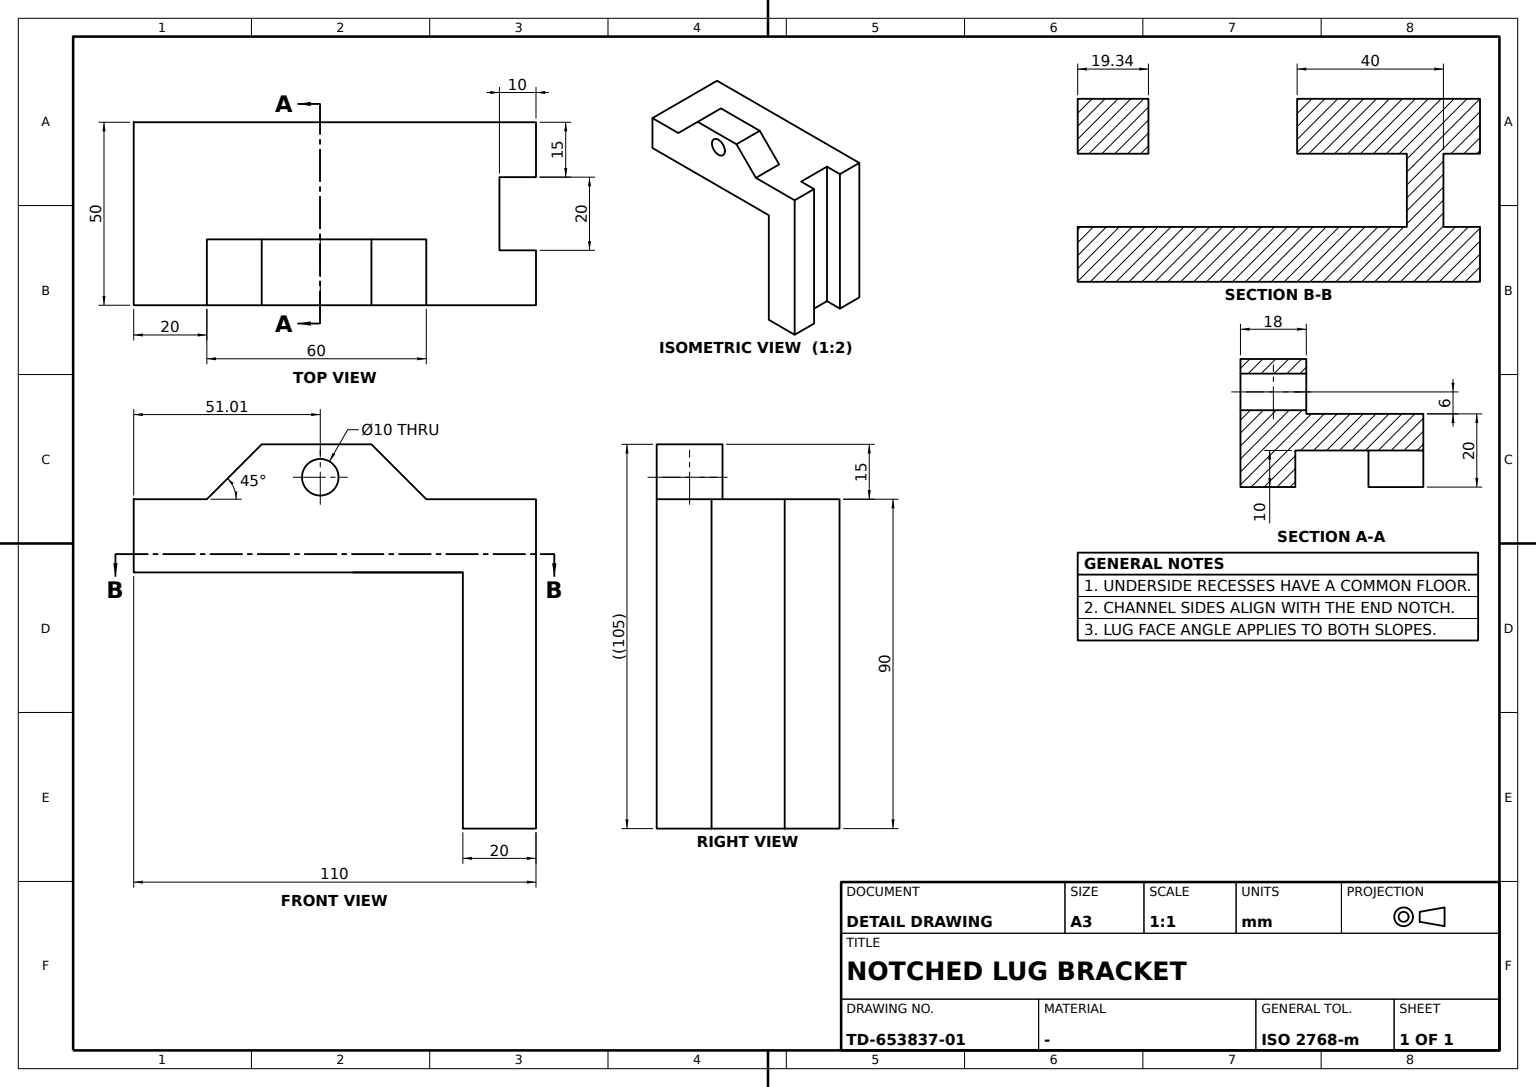
ISO-10303-21;
HEADER;
FILE_DESCRIPTION((''),'2;1');
FILE_NAME('','',(''),(''),'','','');
FILE_SCHEMA(('AUTOMOTIVE_DESIGN'));
ENDSEC;
DATA;
#1=APPLICATION_CONTEXT('');
#2=PRODUCT_CONTEXT('',#1,'mechanical');
#3=PRODUCT('','','',(#2));
#4=PRODUCT_DEFINITION_FORMATION('','',#3);
#5=PRODUCT_DEFINITION_CONTEXT('',#1,'design');
#6=PRODUCT_DEFINITION('','',#4,#5);
#7=PRODUCT_DEFINITION_SHAPE('','',#6);
#8=(LENGTH_UNIT()NAMED_UNIT(*)SI_UNIT(.MILLI.,.METRE.));
#9=(NAMED_UNIT(*)PLANE_ANGLE_UNIT()SI_UNIT($,.RADIAN.));
#10=(NAMED_UNIT(*)SI_UNIT($,.STERADIAN.)SOLID_ANGLE_UNIT());
#11=UNCERTAINTY_MEASURE_WITH_UNIT(LENGTH_MEASURE(1.E-05),#8,'distance_accuracy_value','');
#12=(GEOMETRIC_REPRESENTATION_CONTEXT(3)GLOBAL_UNCERTAINTY_ASSIGNED_CONTEXT((#11))GLOBAL_UNIT_ASSIGNED_CONTEXT((#8,#9,#10))REPRESENTATION_CONTEXT('',''));
#13=CARTESIAN_POINT('',(-33.986597,-12.,6.));
#14=VERTEX_POINT('',#13);
#15=CARTESIAN_POINT('',(-33.986597,-30.,6.));
#16=VERTEX_POINT('',#15);
#17=CARTESIAN_POINT('',(-33.986597,-21.66,6.));
#18=DIRECTION('',(0.,-1.,0.));
#19=VECTOR('',#18,1000.);
#20=LINE('',#17,#19);
#21=EDGE_CURVE('',#14,#16,#20,.T.);
#22=ORIENTED_EDGE('',*,*,#21,.T.);
#23=CARTESIAN_POINT('',(-43.986597,-30.,6.));
#24=VERTEX_POINT('',#23);
#25=CARTESIAN_POINT('',(-38.986597,-30.,6.));
#26=DIRECTION('',(0.,0.,1.));
#27=AXIS2_PLACEMENT_3D('',#25,#18,#26);
#28=CIRCLE('',#27,5.);
#29=EDGE_CURVE('',#16,#24,#28,.T.);
#30=ORIENTED_EDGE('',*,*,#29,.T.);
#31=CARTESIAN_POINT('',(-43.986597,-12.,6.));
#32=VERTEX_POINT('',#31);
#33=CARTESIAN_POINT('',(-43.986597,-21.66,6.));
#34=LINE('',#33,#19);
#35=EDGE_CURVE('',#32,#24,#34,.T.);
#36=ORIENTED_EDGE('',*,*,#35,.F.);
#37=CARTESIAN_POINT('',(-38.986597,-12.,6.));
#38=DIRECTION('',(0.,1.,0.));
#39=DIRECTION('',(-1.,0.,0.));
#40=AXIS2_PLACEMENT_3D('',#37,#38,#39);
#41=CIRCLE('',#40,5.);
#42=EDGE_CURVE('',#32,#14,#41,.T.);
#43=ORIENTED_EDGE('',*,*,#42,.T.);
#44=EDGE_LOOP('',(#22,#30,#36,#43));
#45=FACE_OUTER_BOUND('',#44,.T.);
#46=CARTESIAN_POINT('',(-38.986597,-21.66,6.));
#47=AXIS2_PLACEMENT_3D('',#46,#18,#39);
#48=CYLINDRICAL_SURFACE('',#47,5.);
#49=ADVANCED_FACE('',(#45),#48,.F.);
#50=CARTESIAN_POINT('',(-70.664001,5.,-20.));
#51=VERTEX_POINT('',#50);
#52=CARTESIAN_POINT('',(-90.,5.,-20.));
#53=VERTEX_POINT('',#52);
#54=CARTESIAN_POINT('',(-80.332001,5.,-20.));
#55=VECTOR('',#39,1000.);
#56=LINE('',#54,#55);
#57=EDGE_CURVE('',#51,#53,#56,.T.);
#58=ORIENTED_EDGE('',*,*,#57,.T.);
#59=CARTESIAN_POINT('',(-90.,20.,-20.));
#60=VERTEX_POINT('',#59);
#61=CARTESIAN_POINT('',(-90.,12.5,-20.));
#62=VECTOR('',#38,1000.);
#63=LINE('',#61,#62);
#64=EDGE_CURVE('',#53,#60,#63,.T.);
#65=ORIENTED_EDGE('',*,*,#64,.T.);
#66=CARTESIAN_POINT('',(-70.664001,20.,-20.));
#67=VERTEX_POINT('',#66);
#68=CARTESIAN_POINT('',(-80.332001,20.,-20.));
#69=LINE('',#68,#55);
#70=EDGE_CURVE('',#67,#60,#69,.T.);
#71=ORIENTED_EDGE('',*,*,#70,.F.);
#72=CARTESIAN_POINT('',(-70.664001,12.5,-20.));
#73=LINE('',#72,#19);
#74=EDGE_CURVE('',#67,#51,#73,.T.);
#75=ORIENTED_EDGE('',*,*,#74,.T.);
#76=EDGE_LOOP('',(#58,#65,#71,#75));
#77=FACE_OUTER_BOUND('',#76,.T.);
#78=CARTESIAN_POINT('',(0.,-15.,-20.));
#79=DIRECTION('',(0.,0.,-1.));
#80=AXIS2_PLACEMENT_3D('',#78,#79,#18);
#81=PLANE('',#80);
#82=ADVANCED_FACE('',(#77),#81,.T.);
#83=CARTESIAN_POINT('',(0.,-30.,-20.));
#84=VERTEX_POINT('',#83);
#85=VERTEX_POINT('',#78);
#86=CARTESIAN_POINT('',(0.,-22.5,-20.));
#87=LINE('',#86,#62);
#88=EDGE_CURVE('',#84,#85,#87,.T.);
#89=ORIENTED_EDGE('',*,*,#88,.T.);
#90=CARTESIAN_POINT('',(0.,-15.,-10.));
#91=VERTEX_POINT('',#90);
#92=CARTESIAN_POINT('',(0.,-15.,-15.));
#93=VECTOR('',#26,1000.);
#94=LINE('',#92,#93);
#95=EDGE_CURVE('',#85,#91,#94,.T.);
#96=ORIENTED_EDGE('',*,*,#95,.T.);
#97=CARTESIAN_POINT('',(0.,5.,-10.));
#98=VERTEX_POINT('',#97);
#99=CARTESIAN_POINT('',(0.,-5.,-10.));
#100=LINE('',#99,#62);
#101=EDGE_CURVE('',#91,#98,#100,.T.);
#102=ORIENTED_EDGE('',*,*,#101,.T.);
#103=CARTESIAN_POINT('',(0.,5.,-20.));
#104=VERTEX_POINT('',#103);
#105=CARTESIAN_POINT('',(0.,5.,-15.));
#106=VECTOR('',#79,1000.);
#107=LINE('',#105,#106);
#108=EDGE_CURVE('',#98,#104,#107,.T.);
#109=ORIENTED_EDGE('',*,*,#108,.T.);
#110=CARTESIAN_POINT('',(0.,20.,-20.));
#111=VERTEX_POINT('',#110);
#112=CARTESIAN_POINT('',(0.,12.5,-20.));
#113=LINE('',#112,#62);
#114=EDGE_CURVE('',#104,#111,#113,.T.);
#115=ORIENTED_EDGE('',*,*,#114,.T.);
#116=CARTESIAN_POINT('',(0.,20.,-90.));
#117=VERTEX_POINT('',#116);
#118=CARTESIAN_POINT('',(0.,20.,-55.));
#119=LINE('',#118,#106);
#120=EDGE_CURVE('',#111,#117,#119,.T.);
#121=ORIENTED_EDGE('',*,*,#120,.T.);
#122=CARTESIAN_POINT('',(0.,-30.,-90.));
#123=VERTEX_POINT('',#122);
#124=CARTESIAN_POINT('',(0.,-5.,-90.));
#125=LINE('',#124,#19);
#126=EDGE_CURVE('',#117,#123,#125,.T.);
#127=ORIENTED_EDGE('',*,*,#126,.T.);
#128=CARTESIAN_POINT('',(0.,-30.,-55.));
#129=LINE('',#128,#106);
#130=EDGE_CURVE('',#84,#123,#129,.T.);
#131=ORIENTED_EDGE('',*,*,#130,.F.);
#132=EDGE_LOOP('',(#89,#96,#102,#109,#115,#121,#127,#131));
#133=FACE_OUTER_BOUND('',#132,.T.);
#134=CARTESIAN_POINT('',(0.,0.,0.));
#135=DIRECTION('',(1.,0.,0.));
#136=AXIS2_PLACEMENT_3D('',#134,#135,#38);
#137=PLANE('',#136);
#138=ADVANCED_FACE('',(#133),#137,.F.);
#139=CARTESIAN_POINT('',(10.,5.,0.));
#140=VERTEX_POINT('',#139);
#141=CARTESIAN_POINT('',(10.,5.,-90.));
#142=VERTEX_POINT('',#141);
#143=CARTESIAN_POINT('',(10.,5.,-45.));
#144=LINE('',#143,#106);
#145=EDGE_CURVE('',#140,#142,#144,.T.);
#146=ORIENTED_EDGE('',*,*,#145,.F.);
#147=CARTESIAN_POINT('',(10.,-15.,0.));
#148=VERTEX_POINT('',#147);
#149=CARTESIAN_POINT('',(10.,-5.,0.));
#150=LINE('',#149,#62);
#151=EDGE_CURVE('',#148,#140,#150,.T.);
#152=ORIENTED_EDGE('',*,*,#151,.F.);
#153=CARTESIAN_POINT('',(10.,-15.,-90.));
#154=VERTEX_POINT('',#153);
#155=CARTESIAN_POINT('',(10.,-15.,-45.));
#156=LINE('',#155,#106);
#157=EDGE_CURVE('',#148,#154,#156,.T.);
#158=ORIENTED_EDGE('',*,*,#157,.T.);
#159=CARTESIAN_POINT('',(10.,-5.,-90.));
#160=LINE('',#159,#62);
#161=EDGE_CURVE('',#154,#142,#160,.T.);
#162=ORIENTED_EDGE('',*,*,#161,.T.);
#163=EDGE_LOOP('',(#146,#152,#158,#162));
#164=FACE_OUTER_BOUND('',#163,.T.);
#165=AXIS2_PLACEMENT_3D('',#139,#135,#18);
#166=PLANE('',#165);
#167=ADVANCED_FACE('',(#164),#166,.T.);
#168=CARTESIAN_POINT('',(-30.,20.,-20.));
#169=VERTEX_POINT('',#168);
#170=CARTESIAN_POINT('',(-30.,5.,-20.));
#171=VERTEX_POINT('',#170);
#172=CARTESIAN_POINT('',(-30.,12.5,-20.));
#173=LINE('',#172,#19);
#174=EDGE_CURVE('',#169,#171,#173,.T.);
#175=ORIENTED_EDGE('',*,*,#174,.T.);
#176=CARTESIAN_POINT('',(-30.,5.,-10.));
#177=VERTEX_POINT('',#176);
#178=CARTESIAN_POINT('',(-30.,5.,-15.));
#179=LINE('',#178,#93);
#180=EDGE_CURVE('',#171,#177,#179,.T.);
#181=ORIENTED_EDGE('',*,*,#180,.T.);
#182=CARTESIAN_POINT('',(-30.,20.,-10.));
#183=VERTEX_POINT('',#182);
#184=CARTESIAN_POINT('',(-30.,12.5,-10.));
#185=LINE('',#184,#19);
#186=EDGE_CURVE('',#183,#177,#185,.T.);
#187=ORIENTED_EDGE('',*,*,#186,.F.);
#188=CARTESIAN_POINT('',(-30.,20.,-15.));
#189=LINE('',#188,#106);
#190=EDGE_CURVE('',#183,#169,#189,.T.);
#191=ORIENTED_EDGE('',*,*,#190,.T.);
#192=EDGE_LOOP('',(#175,#181,#187,#191));
#193=FACE_OUTER_BOUND('',#192,.T.);
#194=AXIS2_PLACEMENT_3D('',#168,#135,#26);
#195=PLANE('',#194);
#196=ADVANCED_FACE('',(#193),#195,.F.);
#197=CARTESIAN_POINT('',(-70.,-30.,0.));
#198=VERTEX_POINT('',#197);
#199=CARTESIAN_POINT('',(-55.,-30.,15.));
#200=VERTEX_POINT('',#199);
#201=CARTESIAN_POINT('',(-62.5,-30.,7.5));
#202=DIRECTION('',(0.707106781,0.,0.707106781));
#203=VECTOR('',#202,1000.);
#204=LINE('',#201,#203);
#205=EDGE_CURVE('',#198,#200,#204,.T.);
#206=ORIENTED_EDGE('',*,*,#205,.T.);
#207=CARTESIAN_POINT('',(-55.,-12.,15.));
#208=VERTEX_POINT('',#207);
#209=CARTESIAN_POINT('',(-55.,-21.,15.));
#210=LINE('',#209,#19);
#211=EDGE_CURVE('',#208,#200,#210,.T.);
#212=ORIENTED_EDGE('',*,*,#211,.F.);
#213=CARTESIAN_POINT('',(-70.,-12.,0.));
#214=VERTEX_POINT('',#213);
#215=CARTESIAN_POINT('',(-62.5,-12.,7.5));
#216=DIRECTION('',(-0.707106781,0.,-0.707106781));
#217=VECTOR('',#216,1000.);
#218=LINE('',#215,#217);
#219=EDGE_CURVE('',#208,#214,#218,.T.);
#220=ORIENTED_EDGE('',*,*,#219,.T.);
#221=CARTESIAN_POINT('',(-70.,-21.,0.));
#222=LINE('',#221,#19);
#223=EDGE_CURVE('',#214,#198,#222,.T.);
#224=ORIENTED_EDGE('',*,*,#223,.T.);
#225=EDGE_LOOP('',(#206,#212,#220,#224));
#226=FACE_OUTER_BOUND('',#225,.T.);
#227=CARTESIAN_POINT('',(-70.,-33.6,0.));
#228=DIRECTION('',(0.707106781,0.,-0.707106781));
#229=AXIS2_PLACEMENT_3D('',#227,#228,#38);
#230=PLANE('',#229);
#231=ADVANCED_FACE('',(#226),#230,.F.);
#232=CARTESIAN_POINT('',(-90.,-30.,-20.));
#233=VERTEX_POINT('',#232);
#234=CARTESIAN_POINT('',(-90.,-15.,-20.));
#235=VERTEX_POINT('',#234);
#236=CARTESIAN_POINT('',(-90.,-22.5,-20.));
#237=LINE('',#236,#62);
#238=EDGE_CURVE('',#233,#235,#237,.T.);
#239=ORIENTED_EDGE('',*,*,#238,.F.);
#240=CARTESIAN_POINT('',(-90.,-30.,0.));
#241=VERTEX_POINT('',#240);
#242=CARTESIAN_POINT('',(-90.,-30.,-10.));
#243=LINE('',#242,#106);
#244=EDGE_CURVE('',#241,#233,#243,.T.);
#245=ORIENTED_EDGE('',*,*,#244,.F.);
#246=CARTESIAN_POINT('',(-90.,20.,0.));
#247=VERTEX_POINT('',#246);
#248=CARTESIAN_POINT('',(-90.,-5.,0.));
#249=LINE('',#248,#19);
#250=EDGE_CURVE('',#247,#241,#249,.T.);
#251=ORIENTED_EDGE('',*,*,#250,.F.);
#252=CARTESIAN_POINT('',(-90.,20.,-10.));
#253=LINE('',#252,#93);
#254=EDGE_CURVE('',#60,#247,#253,.T.);
#255=ORIENTED_EDGE('',*,*,#254,.F.);
#256=ORIENTED_EDGE('',*,*,#64,.F.);
#257=CARTESIAN_POINT('',(-90.,5.,-10.));
#258=VERTEX_POINT('',#257);
#259=CARTESIAN_POINT('',(-90.,5.,-15.));
#260=LINE('',#259,#106);
#261=EDGE_CURVE('',#258,#53,#260,.T.);
#262=ORIENTED_EDGE('',*,*,#261,.F.);
#263=CARTESIAN_POINT('',(-90.,-15.,-10.));
#264=VERTEX_POINT('',#263);
#265=CARTESIAN_POINT('',(-90.,-5.,-10.));
#266=LINE('',#265,#62);
#267=EDGE_CURVE('',#264,#258,#266,.T.);
#268=ORIENTED_EDGE('',*,*,#267,.F.);
#269=CARTESIAN_POINT('',(-90.,-15.,-15.));
#270=LINE('',#269,#93);
#271=EDGE_CURVE('',#235,#264,#270,.T.);
#272=ORIENTED_EDGE('',*,*,#271,.F.);
#273=EDGE_LOOP('',(#239,#245,#251,#255,#256,#262,#268,#272));
#274=FACE_OUTER_BOUND('',#273,.T.);
#275=CARTESIAN_POINT('',(-90.,0.,0.));
#276=AXIS2_PLACEMENT_3D('',#275,#135,#38);
#277=PLANE('',#276);
#278=ADVANCED_FACE('',(#274),#277,.F.);
#279=CARTESIAN_POINT('',(20.,-30.,0.));
#280=VERTEX_POINT('',#279);
#281=CARTESIAN_POINT('',(20.,-15.,0.));
#282=VERTEX_POINT('',#281);
#283=CARTESIAN_POINT('',(20.,-22.5,0.));
#284=LINE('',#283,#62);
#285=EDGE_CURVE('',#280,#282,#284,.T.);
#286=ORIENTED_EDGE('',*,*,#285,.F.);
#287=CARTESIAN_POINT('',(20.,-30.,-90.));
#288=VERTEX_POINT('',#287);
#289=CARTESIAN_POINT('',(20.,-30.,-45.));
#290=LINE('',#289,#106);
#291=EDGE_CURVE('',#280,#288,#290,.T.);
#292=ORIENTED_EDGE('',*,*,#291,.T.);
#293=CARTESIAN_POINT('',(20.,-15.,-90.));
#294=VERTEX_POINT('',#293);
#295=CARTESIAN_POINT('',(20.,-22.5,-90.));
#296=LINE('',#295,#62);
#297=EDGE_CURVE('',#288,#294,#296,.T.);
#298=ORIENTED_EDGE('',*,*,#297,.T.);
#299=CARTESIAN_POINT('',(20.,-15.,-45.));
#300=LINE('',#299,#106);
#301=EDGE_CURVE('',#282,#294,#300,.T.);
#302=ORIENTED_EDGE('',*,*,#301,.F.);
#303=EDGE_LOOP('',(#286,#292,#298,#302));
#304=FACE_OUTER_BOUND('',#303,.T.);
#305=AXIS2_PLACEMENT_3D('',#281,#135,#18);
#306=PLANE('',#305);
#307=ADVANCED_FACE('',(#304),#306,.T.);
#308=CARTESIAN_POINT('',(-45.,-15.,-20.));
#309=LINE('',#308,#55);
#310=EDGE_CURVE('',#85,#235,#309,.T.);
#311=ORIENTED_EDGE('',*,*,#310,.F.);
#312=ORIENTED_EDGE('',*,*,#88,.F.);
#313=CARTESIAN_POINT('',(-45.,-30.,-20.));
#314=LINE('',#313,#55);
#315=EDGE_CURVE('',#84,#233,#314,.T.);
#316=ORIENTED_EDGE('',*,*,#315,.T.);
#317=ORIENTED_EDGE('',*,*,#238,.T.);
#318=EDGE_LOOP('',(#311,#312,#316,#317));
#319=FACE_OUTER_BOUND('',#318,.T.);
#320=ADVANCED_FACE('',(#319),#81,.T.);
#321=CARTESIAN_POINT('',(20.,5.,0.));
#322=VERTEX_POINT('',#321);
#323=CARTESIAN_POINT('',(20.,5.,-90.));
#324=VERTEX_POINT('',#323);
#325=CARTESIAN_POINT('',(20.,5.,-45.));
#326=LINE('',#325,#106);
#327=EDGE_CURVE('',#322,#324,#326,.T.);
#328=ORIENTED_EDGE('',*,*,#327,.F.);
#329=CARTESIAN_POINT('',(15.,5.,0.));
#330=VECTOR('',#135,1000.);
#331=LINE('',#329,#330);
#332=EDGE_CURVE('',#140,#322,#331,.T.);
#333=ORIENTED_EDGE('',*,*,#332,.F.);
#334=ORIENTED_EDGE('',*,*,#145,.T.);
#335=CARTESIAN_POINT('',(15.,5.,-90.));
#336=LINE('',#335,#330);
#337=EDGE_CURVE('',#142,#324,#336,.T.);
#338=ORIENTED_EDGE('',*,*,#337,.T.);
#339=EDGE_LOOP('',(#328,#333,#334,#338));
#340=FACE_OUTER_BOUND('',#339,.T.);
#341=AXIS2_PLACEMENT_3D('',#103,#18,#26);
#342=PLANE('',#341);
#343=ADVANCED_FACE('',(#340),#342,.T.);
#344=CARTESIAN_POINT('',(-25.,-30.,15.));
#345=VERTEX_POINT('',#344);
#346=CARTESIAN_POINT('',(-25.,-12.,15.));
#347=VERTEX_POINT('',#346);
#348=CARTESIAN_POINT('',(-25.,-21.,15.));
#349=LINE('',#348,#62);
#350=EDGE_CURVE('',#345,#347,#349,.T.);
#351=ORIENTED_EDGE('',*,*,#350,.T.);
#352=CARTESIAN_POINT('',(-40.,-12.,15.));
#353=LINE('',#352,#55);
#354=EDGE_CURVE('',#347,#208,#353,.T.);
#355=ORIENTED_EDGE('',*,*,#354,.T.);
#356=ORIENTED_EDGE('',*,*,#211,.T.);
#357=CARTESIAN_POINT('',(-40.,-30.,15.));
#358=LINE('',#357,#330);
#359=EDGE_CURVE('',#200,#345,#358,.T.);
#360=ORIENTED_EDGE('',*,*,#359,.T.);
#361=EDGE_LOOP('',(#351,#355,#356,#360));
#362=FACE_OUTER_BOUND('',#361,.T.);
#363=CARTESIAN_POINT('',(0.,0.,15.));
#364=AXIS2_PLACEMENT_3D('',#363,#26,#135);
#365=PLANE('',#364);
#366=ADVANCED_FACE('',(#362),#365,.T.);
#367=ORIENTED_EDGE('',*,*,#180,.F.);
#368=CARTESIAN_POINT('',(-15.,5.,-20.));
#369=LINE('',#368,#55);
#370=EDGE_CURVE('',#104,#171,#369,.T.);
#371=ORIENTED_EDGE('',*,*,#370,.F.);
#372=ORIENTED_EDGE('',*,*,#108,.F.);
#373=CARTESIAN_POINT('',(-15.,5.,-10.));
#374=LINE('',#373,#55);
#375=EDGE_CURVE('',#98,#177,#374,.T.);
#376=ORIENTED_EDGE('',*,*,#375,.T.);
#377=EDGE_LOOP('',(#367,#371,#372,#376));
#378=FACE_OUTER_BOUND('',#377,.T.);
#379=ADVANCED_FACE('',(#378),#342,.T.);
#380=CARTESIAN_POINT('',(20.,20.,-90.));
#381=VERTEX_POINT('',#380);
#382=CARTESIAN_POINT('',(10.,20.,-90.));
#383=LINE('',#382,#55);
#384=EDGE_CURVE('',#381,#117,#383,.T.);
#385=ORIENTED_EDGE('',*,*,#384,.F.);
#386=CARTESIAN_POINT('',(20.,12.5,-90.));
#387=LINE('',#386,#62);
#388=EDGE_CURVE('',#324,#381,#387,.T.);
#389=ORIENTED_EDGE('',*,*,#388,.F.);
#390=ORIENTED_EDGE('',*,*,#337,.F.);
#391=ORIENTED_EDGE('',*,*,#161,.F.);
#392=CARTESIAN_POINT('',(15.,-15.,-90.));
#393=LINE('',#392,#55);
#394=EDGE_CURVE('',#294,#154,#393,.T.);
#395=ORIENTED_EDGE('',*,*,#394,.F.);
#396=ORIENTED_EDGE('',*,*,#297,.F.);
#397=CARTESIAN_POINT('',(10.,-30.,-90.));
#398=LINE('',#397,#330);
#399=EDGE_CURVE('',#123,#288,#398,.T.);
#400=ORIENTED_EDGE('',*,*,#399,.F.);
#401=ORIENTED_EDGE('',*,*,#126,.F.);
#402=EDGE_LOOP('',(#385,#389,#390,#391,#395,#396,#400,#401));
#403=FACE_OUTER_BOUND('',#402,.T.);
#404=CARTESIAN_POINT('',(0.,0.,-90.));
#405=AXIS2_PLACEMENT_3D('',#404,#26,#38);
#406=PLANE('',#405);
#407=ADVANCED_FACE('',(#403),#406,.F.);
#408=CARTESIAN_POINT('',(-10.,-12.,0.));
#409=VERTEX_POINT('',#408);
#410=CARTESIAN_POINT('',(-17.5,-12.,7.5));
#411=DIRECTION('',(-0.707106781,0.,0.707106781));
#412=VECTOR('',#411,1000.);
#413=LINE('',#410,#412);
#414=EDGE_CURVE('',#409,#347,#413,.T.);
#415=ORIENTED_EDGE('',*,*,#414,.T.);
#416=ORIENTED_EDGE('',*,*,#350,.F.);
#417=CARTESIAN_POINT('',(-10.,-30.,0.));
#418=VERTEX_POINT('',#417);
#419=CARTESIAN_POINT('',(-17.5,-30.,7.5));
#420=VECTOR('',#228,1000.);
#421=LINE('',#419,#420);
#422=EDGE_CURVE('',#345,#418,#421,.T.);
#423=ORIENTED_EDGE('',*,*,#422,.T.);
#424=CARTESIAN_POINT('',(-10.,-21.,0.));
#425=LINE('',#424,#62);
#426=EDGE_CURVE('',#418,#409,#425,.T.);
#427=ORIENTED_EDGE('',*,*,#426,.T.);
#428=EDGE_LOOP('',(#415,#416,#423,#427));
#429=FACE_OUTER_BOUND('',#428,.T.);
#430=CARTESIAN_POINT('',(-10.,-8.4,0.));
#431=AXIS2_PLACEMENT_3D('',#430,#216,#18);
#432=PLANE('',#431);
#433=ADVANCED_FACE('',(#429),#432,.F.);
#434=EDGE_CURVE('',#24,#16,#28,.T.);
#435=ORIENTED_EDGE('',*,*,#434,.T.);
#436=ORIENTED_EDGE('',*,*,#21,.F.);
#437=EDGE_CURVE('',#14,#32,#41,.T.);
#438=ORIENTED_EDGE('',*,*,#437,.T.);
#439=ORIENTED_EDGE('',*,*,#35,.T.);
#440=EDGE_LOOP('',(#435,#436,#438,#439));
#441=FACE_OUTER_BOUND('',#440,.T.);
#442=ADVANCED_FACE('',(#441),#48,.F.);
#443=CARTESIAN_POINT('',(-70.664001,20.,-10.));
#444=VERTEX_POINT('',#443);
#445=CARTESIAN_POINT('',(-50.332001,20.,-10.));
#446=LINE('',#445,#330);
#447=EDGE_CURVE('',#444,#183,#446,.T.);
#448=ORIENTED_EDGE('',*,*,#447,.T.);
#449=ORIENTED_EDGE('',*,*,#186,.T.);
#450=ORIENTED_EDGE('',*,*,#375,.F.);
#451=ORIENTED_EDGE('',*,*,#101,.F.);
#452=CARTESIAN_POINT('',(-45.,-15.,-10.));
#453=LINE('',#452,#55);
#454=EDGE_CURVE('',#91,#264,#453,.T.);
#455=ORIENTED_EDGE('',*,*,#454,.T.);
#456=ORIENTED_EDGE('',*,*,#267,.T.);
#457=CARTESIAN_POINT('',(-70.664001,5.,-10.));
#458=VERTEX_POINT('',#457);
#459=CARTESIAN_POINT('',(-80.332001,5.,-10.));
#460=LINE('',#459,#55);
#461=EDGE_CURVE('',#458,#258,#460,.T.);
#462=ORIENTED_EDGE('',*,*,#461,.F.);
#463=CARTESIAN_POINT('',(-70.664001,12.5,-10.));
#464=LINE('',#463,#19);
#465=EDGE_CURVE('',#444,#458,#464,.T.);
#466=ORIENTED_EDGE('',*,*,#465,.F.);
#467=EDGE_LOOP('',(#448,#449,#450,#451,#455,#456,#462,#466));
#468=FACE_OUTER_BOUND('',#467,.T.);
#469=AXIS2_PLACEMENT_3D('',#97,#79,#18);
#470=PLANE('',#469);
#471=ADVANCED_FACE('',(#468),#470,.T.);
#472=ORIENTED_EDGE('',*,*,#261,.T.);
#473=ORIENTED_EDGE('',*,*,#57,.F.);
#474=CARTESIAN_POINT('',(-70.664001,5.,-15.));
#475=LINE('',#474,#93);
#476=EDGE_CURVE('',#51,#458,#475,.T.);
#477=ORIENTED_EDGE('',*,*,#476,.T.);
#478=ORIENTED_EDGE('',*,*,#461,.T.);
#479=EDGE_LOOP('',(#472,#473,#477,#478));
#480=FACE_OUTER_BOUND('',#479,.T.);
#481=ADVANCED_FACE('',(#480),#342,.T.);
#482=ORIENTED_EDGE('',*,*,#254,.T.);
#483=CARTESIAN_POINT('',(20.,20.,0.));
#484=VERTEX_POINT('',#483);
#485=CARTESIAN_POINT('',(-35.,20.,0.));
#486=LINE('',#485,#55);
#487=EDGE_CURVE('',#484,#247,#486,.T.);
#488=ORIENTED_EDGE('',*,*,#487,.F.);
#489=CARTESIAN_POINT('',(20.,20.,-45.));
#490=LINE('',#489,#106);
#491=EDGE_CURVE('',#484,#381,#490,.T.);
#492=ORIENTED_EDGE('',*,*,#491,.T.);
#493=ORIENTED_EDGE('',*,*,#384,.T.);
#494=ORIENTED_EDGE('',*,*,#120,.F.);
#495=CARTESIAN_POINT('',(-15.,20.,-20.));
#496=LINE('',#495,#55);
#497=EDGE_CURVE('',#111,#169,#496,.T.);
#498=ORIENTED_EDGE('',*,*,#497,.T.);
#499=ORIENTED_EDGE('',*,*,#190,.F.);
#500=ORIENTED_EDGE('',*,*,#447,.F.);
#501=CARTESIAN_POINT('',(-70.664001,20.,-15.));
#502=LINE('',#501,#93);
#503=EDGE_CURVE('',#67,#444,#502,.T.);
#504=ORIENTED_EDGE('',*,*,#503,.F.);
#505=ORIENTED_EDGE('',*,*,#70,.T.);
#506=EDGE_LOOP('',(#482,#488,#492,#493,#494,#498,#499,#500,#504,#505));
#507=FACE_OUTER_BOUND('',#506,.T.);
#508=CARTESIAN_POINT('',(0.,20.,0.));
#509=AXIS2_PLACEMENT_3D('',#508,#38,#79);
#510=PLANE('',#509);
#511=ADVANCED_FACE('',(#507),#510,.T.);
#512=ORIENTED_EDGE('',*,*,#437,.F.);
#513=ORIENTED_EDGE('',*,*,#42,.F.);
#514=EDGE_LOOP('',(#512,#513));
#515=FACE_BOUND('',#514,.T.);
#516=ORIENTED_EDGE('',*,*,#219,.F.);
#517=ORIENTED_EDGE('',*,*,#354,.F.);
#518=ORIENTED_EDGE('',*,*,#414,.F.);
#519=CARTESIAN_POINT('',(-40.,-12.,0.));
#520=LINE('',#519,#55);
#521=EDGE_CURVE('',#409,#214,#520,.T.);
#522=ORIENTED_EDGE('',*,*,#521,.T.);
#523=EDGE_LOOP('',(#516,#517,#518,#522));
#524=FACE_OUTER_BOUND('',#523,.T.);
#525=AXIS2_PLACEMENT_3D('',#213,#18,#135);
#526=PLANE('',#525);
#527=ADVANCED_FACE('',(#515,#524),#526,.F.);
#528=ORIENTED_EDGE('',*,*,#422,.F.);
#529=ORIENTED_EDGE('',*,*,#359,.F.);
#530=ORIENTED_EDGE('',*,*,#205,.F.);
#531=CARTESIAN_POINT('',(-80.,-30.,0.));
#532=LINE('',#531,#55);
#533=EDGE_CURVE('',#198,#241,#532,.T.);
#534=ORIENTED_EDGE('',*,*,#533,.T.);
#535=ORIENTED_EDGE('',*,*,#244,.T.);
#536=ORIENTED_EDGE('',*,*,#315,.F.);
#537=ORIENTED_EDGE('',*,*,#130,.T.);
#538=ORIENTED_EDGE('',*,*,#399,.T.);
#539=ORIENTED_EDGE('',*,*,#291,.F.);
#540=CARTESIAN_POINT('',(10.,-30.,0.));
#541=LINE('',#540,#330);
#542=EDGE_CURVE('',#418,#280,#541,.T.);
#543=ORIENTED_EDGE('',*,*,#542,.F.);
#544=EDGE_LOOP('',(#528,#529,#530,#534,#535,#536,#537,#538,#539,#543));
#545=FACE_OUTER_BOUND('',#544,.T.);
#546=ORIENTED_EDGE('',*,*,#29,.F.);
#547=ORIENTED_EDGE('',*,*,#434,.F.);
#548=EDGE_LOOP('',(#546,#547));
#549=FACE_BOUND('',#548,.T.);
#550=AXIS2_PLACEMENT_3D('',#83,#18,#26);
#551=PLANE('',#550);
#552=ADVANCED_FACE('',(#545,#549),#551,.T.);
#553=ORIENTED_EDGE('',*,*,#503,.T.);
#554=ORIENTED_EDGE('',*,*,#465,.T.);
#555=ORIENTED_EDGE('',*,*,#476,.F.);
#556=ORIENTED_EDGE('',*,*,#74,.F.);
#557=EDGE_LOOP('',(#553,#554,#555,#556));
#558=FACE_OUTER_BOUND('',#557,.T.);
#559=AXIS2_PLACEMENT_3D('',#443,#39,#79);
#560=PLANE('',#559);
#561=ADVANCED_FACE('',(#558),#560,.F.);
#562=ORIENTED_EDGE('',*,*,#542,.T.);
#563=ORIENTED_EDGE('',*,*,#285,.T.);
#564=CARTESIAN_POINT('',(15.,-15.,0.));
#565=LINE('',#564,#55);
#566=EDGE_CURVE('',#282,#148,#565,.T.);
#567=ORIENTED_EDGE('',*,*,#566,.T.);
#568=ORIENTED_EDGE('',*,*,#151,.T.);
#569=ORIENTED_EDGE('',*,*,#332,.T.);
#570=CARTESIAN_POINT('',(20.,12.5,0.));
#571=LINE('',#570,#62);
#572=EDGE_CURVE('',#322,#484,#571,.T.);
#573=ORIENTED_EDGE('',*,*,#572,.T.);
#574=ORIENTED_EDGE('',*,*,#487,.T.);
#575=ORIENTED_EDGE('',*,*,#250,.T.);
#576=ORIENTED_EDGE('',*,*,#533,.F.);
#577=ORIENTED_EDGE('',*,*,#223,.F.);
#578=ORIENTED_EDGE('',*,*,#521,.F.);
#579=ORIENTED_EDGE('',*,*,#426,.F.);
#580=EDGE_LOOP('',(#562,#563,#567,#568,#569,#573,#574,#575,#576,#577,#578,#579));
#581=FACE_OUTER_BOUND('',#580,.T.);
#582=CARTESIAN_POINT('',(0.,-30.,0.));
#583=AXIS2_PLACEMENT_3D('',#582,#26,#38);
#584=PLANE('',#583);
#585=ADVANCED_FACE('',(#581),#584,.T.);
#586=ORIENTED_EDGE('',*,*,#301,.T.);
#587=ORIENTED_EDGE('',*,*,#394,.T.);
#588=ORIENTED_EDGE('',*,*,#157,.F.);
#589=ORIENTED_EDGE('',*,*,#566,.F.);
#590=EDGE_LOOP('',(#586,#587,#588,#589));
#591=FACE_OUTER_BOUND('',#590,.T.);
#592=AXIS2_PLACEMENT_3D('',#90,#38,#79);
#593=PLANE('',#592);
#594=ADVANCED_FACE('',(#591),#593,.T.);
#595=ORIENTED_EDGE('',*,*,#271,.T.);
#596=ORIENTED_EDGE('',*,*,#454,.F.);
#597=ORIENTED_EDGE('',*,*,#95,.F.);
#598=ORIENTED_EDGE('',*,*,#310,.T.);
#599=EDGE_LOOP('',(#595,#596,#597,#598));
#600=FACE_OUTER_BOUND('',#599,.T.);
#601=ADVANCED_FACE('',(#600),#593,.T.);
#602=ORIENTED_EDGE('',*,*,#572,.F.);
#603=ORIENTED_EDGE('',*,*,#327,.T.);
#604=ORIENTED_EDGE('',*,*,#388,.T.);
#605=ORIENTED_EDGE('',*,*,#491,.F.);
#606=EDGE_LOOP('',(#602,#603,#604,#605));
#607=FACE_OUTER_BOUND('',#606,.T.);
#608=ADVANCED_FACE('',(#607),#306,.T.);
#609=ORIENTED_EDGE('',*,*,#370,.T.);
#610=ORIENTED_EDGE('',*,*,#174,.F.);
#611=ORIENTED_EDGE('',*,*,#497,.F.);
#612=ORIENTED_EDGE('',*,*,#114,.F.);
#613=EDGE_LOOP('',(#609,#610,#611,#612));
#614=FACE_OUTER_BOUND('',#613,.T.);
#615=ADVANCED_FACE('',(#614),#81,.T.);
#616=CLOSED_SHELL('',(#49,#82,#138,#167,#196,#231,#278,#307,#320,#343,#366,#379,#407,#433,#442,#471,#481,#511,#527,#552,#561,#585,#594,#601,#608,#615));
#617=MANIFOLD_SOLID_BREP('',#616);
#618=ADVANCED_BREP_SHAPE_REPRESENTATION('',(#617),#12);
#619=SHAPE_DEFINITION_REPRESENTATION(#7,#618);
ENDSEC;
END-ISO-10303-21;
